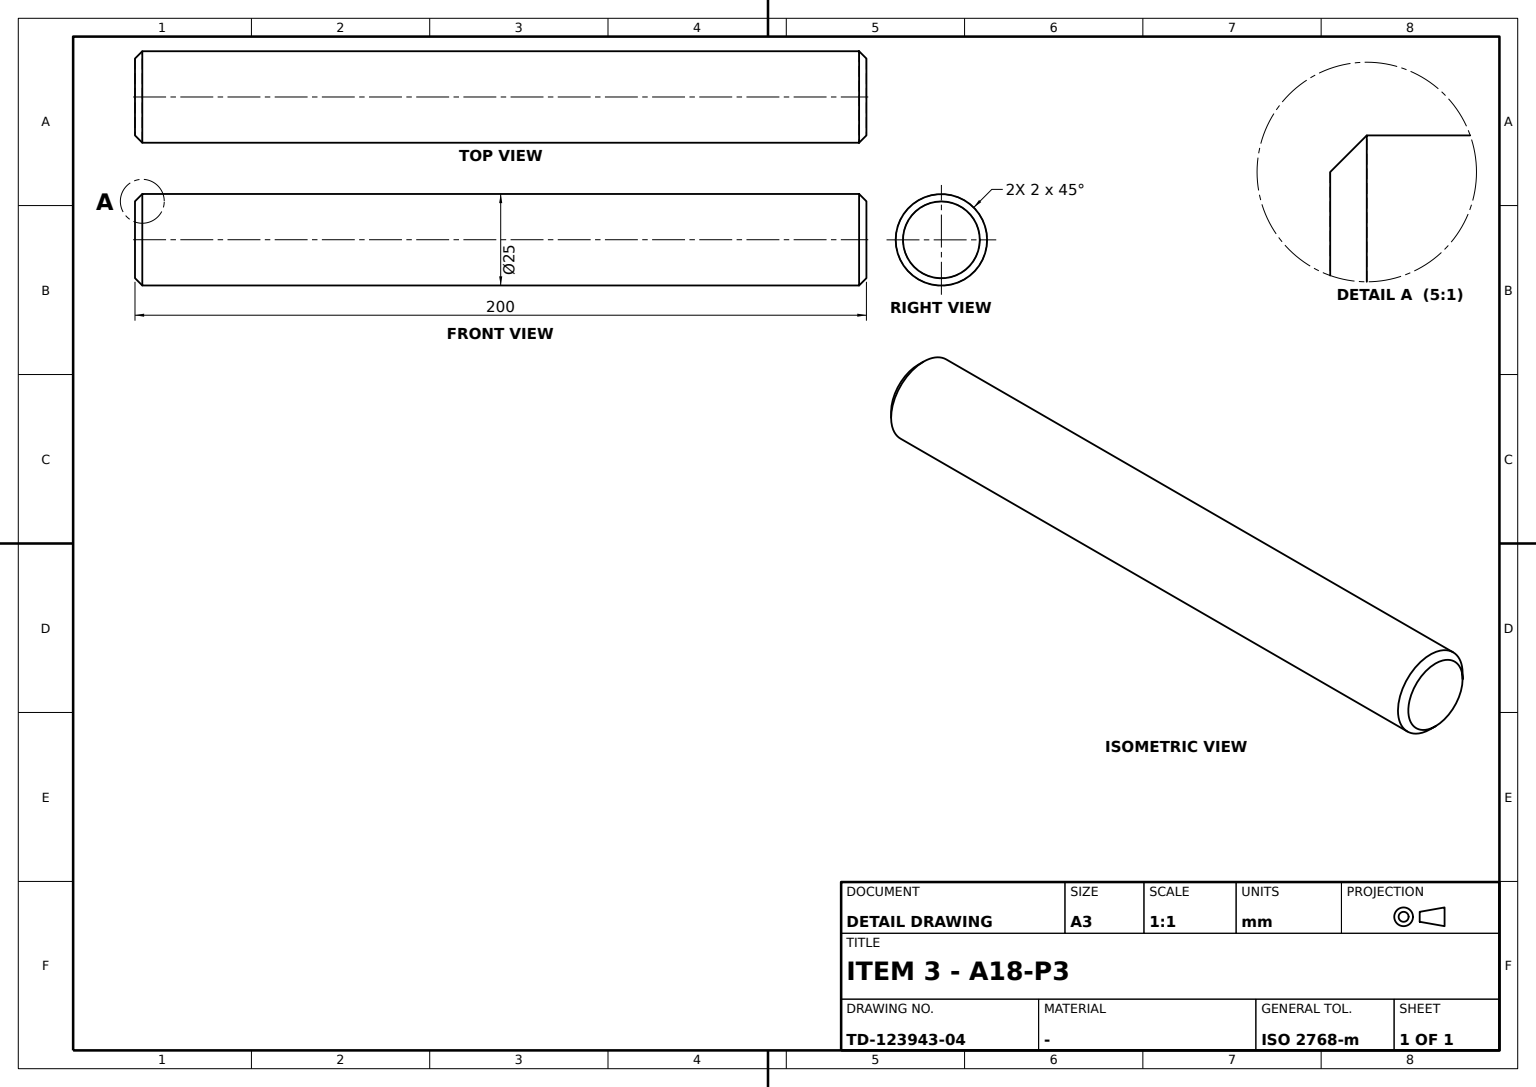
ISO-10303-21;
HEADER;
FILE_DESCRIPTION((''),'2;1');
FILE_NAME('','',(''),(''),'','','');
FILE_SCHEMA(('AUTOMOTIVE_DESIGN'));
ENDSEC;
DATA;
#1=APPLICATION_CONTEXT('');
#2=PRODUCT_CONTEXT('',#1,'mechanical');
#3=PRODUCT('','','',(#2));
#4=PRODUCT_DEFINITION_FORMATION('','',#3);
#5=PRODUCT_DEFINITION_CONTEXT('',#1,'design');
#6=PRODUCT_DEFINITION('','',#4,#5);
#7=PRODUCT_DEFINITION_SHAPE('','',#6);
#8=(LENGTH_UNIT()NAMED_UNIT(*)SI_UNIT(.MILLI.,.METRE.));
#9=(NAMED_UNIT(*)PLANE_ANGLE_UNIT()SI_UNIT($,.RADIAN.));
#10=(NAMED_UNIT(*)SI_UNIT($,.STERADIAN.)SOLID_ANGLE_UNIT());
#11=UNCERTAINTY_MEASURE_WITH_UNIT(LENGTH_MEASURE(0.005),#8,'distance_accuracy_value','');
#12=(GEOMETRIC_REPRESENTATION_CONTEXT(3)GLOBAL_UNCERTAINTY_ASSIGNED_CONTEXT((#11))GLOBAL_UNIT_ASSIGNED_CONTEXT((#8,#9,#10))REPRESENTATION_CONTEXT('',''));
#13=CARTESIAN_POINT('',(-10.5,0.,0.));
#14=VERTEX_POINT('',#13);
#15=CARTESIAN_POINT('',(0.,0.,0.));
#16=DIRECTION('',(0.,0.,-1.));
#17=DIRECTION('',(-1.,0.,0.));
#18=AXIS2_PLACEMENT_3D('',#15,#16,#17);
#19=CIRCLE('',#18,10.5);
#20=EDGE_CURVE('',#14,#14,#19,.T.);
#21=ORIENTED_EDGE('',*,*,#20,.F.);
#22=EDGE_LOOP('',(#21));
#23=FACE_BOUND('',#22,.T.);
#24=CARTESIAN_POINT('',(0.,-12.5,2.));
#25=VERTEX_POINT('',#24);
#26=CARTESIAN_POINT('',(0.,0.,2.));
#27=DIRECTION('',(0.,0.,1.));
#28=DIRECTION('',(0.,-1.,0.));
#29=AXIS2_PLACEMENT_3D('',#26,#27,#28);
#30=CIRCLE('',#29,12.5);
#31=EDGE_CURVE('',#25,#25,#30,.F.);
#32=ORIENTED_EDGE('',*,*,#31,.T.);
#33=EDGE_LOOP('',(#32));
#34=FACE_BOUND('',#33,.T.);
#35=CARTESIAN_POINT('',(0.,0.,-10.5));
#36=DIRECTION('',(-0.479425539,-0.877582562,0.));
#37=AXIS2_PLACEMENT_3D('',#35,#27,#36);
#38=CONICAL_SURFACE('',#37,0.,0.785398163);
#39=ADVANCED_FACE('',(#23,#34),#38,.T.);
#40=ORIENTED_EDGE('',*,*,#20,.T.);
#41=EDGE_LOOP('',(#40));
#42=FACE_BOUND('',#41,.T.);
#43=CARTESIAN_POINT('',(0.,12.5,0.));
#44=DIRECTION('',(1.,0.,0.));
#45=AXIS2_PLACEMENT_3D('',#43,#16,#44);
#46=PLANE('',#45);
#47=ADVANCED_FACE('',(#42),#46,.T.);
#48=CARTESIAN_POINT('',(0.,12.5,198.));
#49=VERTEX_POINT('',#48);
#50=CARTESIAN_POINT('',(0.,0.,198.));
#51=DIRECTION('',(0.,1.,0.));
#52=AXIS2_PLACEMENT_3D('',#50,#16,#51);
#53=CIRCLE('',#52,12.5);
#54=EDGE_CURVE('',#49,#49,#53,.T.);
#55=ORIENTED_EDGE('',*,*,#54,.F.);
#56=EDGE_LOOP('',(#55));
#57=FACE_BOUND('',#56,.T.);
#58=CARTESIAN_POINT('',(-10.5,0.,200.));
#59=VERTEX_POINT('',#58);
#60=CARTESIAN_POINT('',(0.,0.,200.));
#61=AXIS2_PLACEMENT_3D('',#60,#16,#17);
#62=CIRCLE('',#61,10.5);
#63=EDGE_CURVE('',#59,#59,#62,.T.);
#64=ORIENTED_EDGE('',*,*,#63,.T.);
#65=EDGE_LOOP('',(#64));
#66=FACE_BOUND('',#65,.T.);
#67=CARTESIAN_POINT('',(0.,0.,210.5));
#68=DIRECTION('',(0.479425539,0.877582562,0.));
#69=AXIS2_PLACEMENT_3D('',#67,#16,#68);
#70=CONICAL_SURFACE('',#69,0.,0.785398163);
#71=ADVANCED_FACE('',(#57,#66),#70,.T.);
#72=ORIENTED_EDGE('',*,*,#54,.T.);
#73=EDGE_LOOP('',(#72));
#74=FACE_BOUND('',#73,.T.);
#75=ORIENTED_EDGE('',*,*,#31,.F.);
#76=EDGE_LOOP('',(#75));
#77=FACE_BOUND('',#76,.T.);
#78=CARTESIAN_POINT('',(0.,0.,100.));
#79=AXIS2_PLACEMENT_3D('',#78,#16,#44);
#80=CYLINDRICAL_SURFACE('',#79,12.5);
#81=ADVANCED_FACE('',(#74,#77),#80,.T.);
#82=ORIENTED_EDGE('',*,*,#63,.F.);
#83=EDGE_LOOP('',(#82));
#84=FACE_BOUND('',#83,.T.);
#85=AXIS2_PLACEMENT_3D('',#60,#16,#44);
#86=PLANE('',#85);
#87=ADVANCED_FACE('',(#84),#86,.F.);
#88=CLOSED_SHELL('',(#39,#47,#71,#81,#87));
#89=MANIFOLD_SOLID_BREP('',#88);
#90=ADVANCED_BREP_SHAPE_REPRESENTATION('',(#89),#12);
#91=SHAPE_DEFINITION_REPRESENTATION(#7,#90);
ENDSEC;
END-ISO-10303-21;
